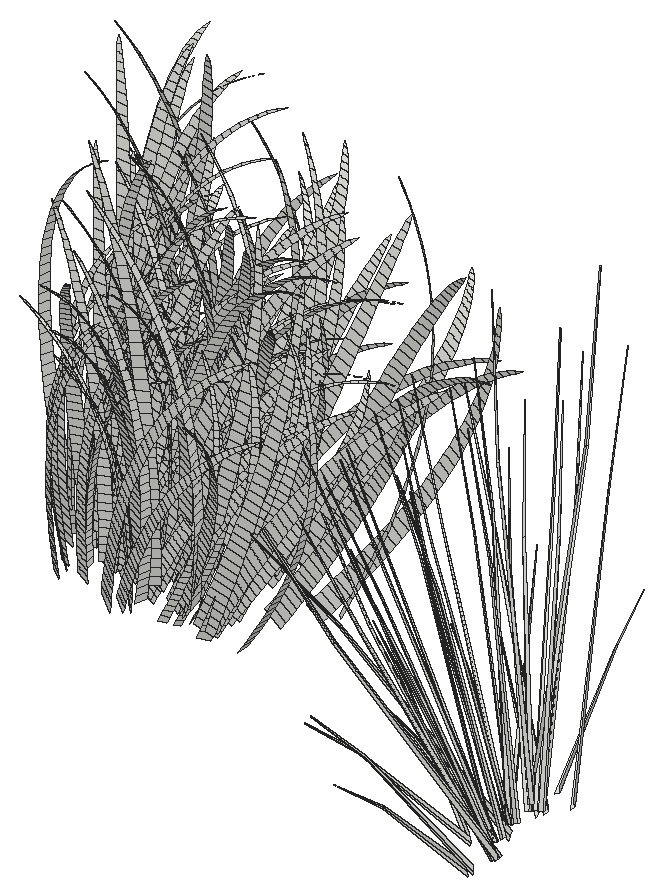
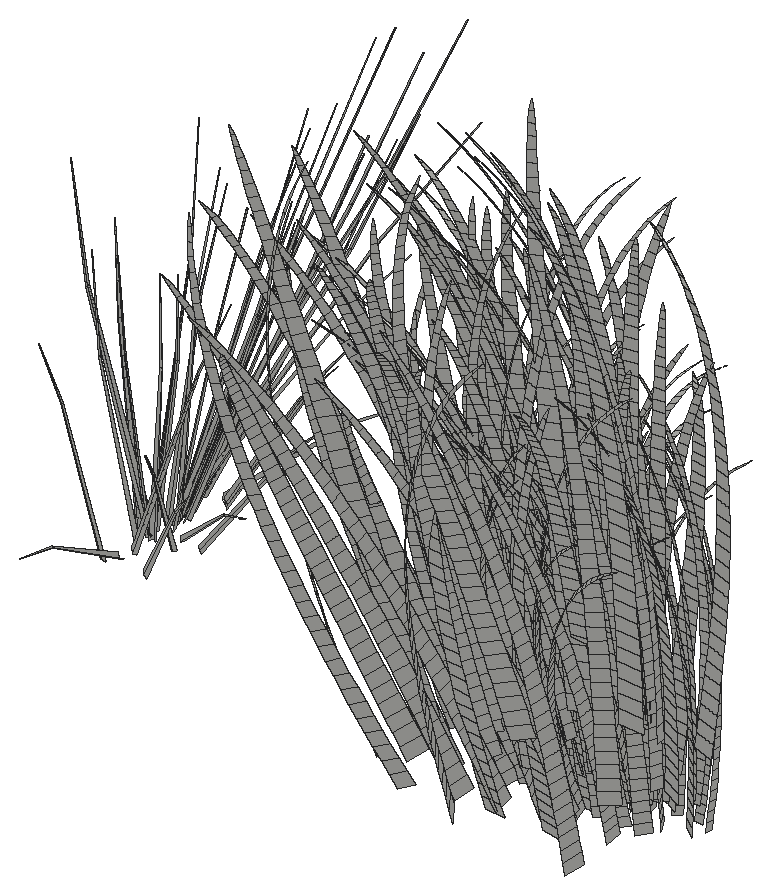
# SketchUp Ruby script. Lengths in inches.
U = 1.inch
M = Sketchup.active_model
def pt(a) = Geom::Point3d.new(a.map { |v| v * U })
def face(e, loops, mat)
  f = e.add_face(loops[0].map { |a| pt(a) })
  loops[1..].each { |l| e.add_face(l.map { |a| pt(a) }).erase! }
  f.material = f.back_material = mat if mat
  f
end
# faces: each face lists its corners as indices into pts; further lists are holes
def faces(e, pts, list, mat = nil) = list.each { |f| face(e, (f[0].is_a?(Array) ? f : [f]).map { |l| l.map { |i| pts[i] } }, mat) }
# xy, xz, yz: faces in a plane at the given z, y or x. An outline is a flat list of corners, or four numbers for a rectangle; further outlines are holes
def ring(l) = l.size == 4 ? [[l[0], l[1]], [l[2], l[1]], [l[2], l[3]], [l[0], l[3]]] : l.each_slice(2).to_a
def flat(e, list, mat, &to3) = list.each { |f| face(e, (f[0].is_a?(Array) ? f : [f]).map { |l| ring(l).map { |u, v| to3.(u, v) } }, mat) }
def xy(e, z, list, mat = nil) = flat(e, list, mat) { |x, y| [x, y, z] }
def xz(e, y, list, mat = nil) = flat(e, list, mat) { |x, z| [x, y, z] }
def yz(e, x, list, mat = nil) = flat(e, list, mat) { |y, z| [x, y, z] }
def lines(e, pts, list) = list.each { |a, b| e.add_line(pt(pts[a]), pt(pts[b])) }
# prism: a flat outline (further loops are holes) pulled along v
def prism(e, loops, v, mat = nil)
  f = face(e, loops, mat); d = Geom::Vector3d.new(v.map { |x| x * U })
  f.pushpull(f.normal.samedirection?(d) ? d.length : -d.length)
end
def box(e, o, s, mat = nil) = prism(e, [[o, [o[0] + s[0], o[1], o[2]], [o[0] + s[0], o[1] + s[1], o[2]], [o[0], o[1] + s[1], o[2]]]], [0, 0, s[2]], mat)
def at(x, y, z, deg = 0) = Geom::Transformation.translation(pt([x, y, z])) * Geom::Transformation.rotation(ORIGIN, Z_AXIS, deg.degrees)
def axes(o, x, y, z) = Geom::Transformation.new([*x, 0, *y, 0, *z, 0, *pt(o).to_a, 1])
def part(name) = M.definitions.add(name)
# library, detail: a bought-in or finely detailed component or shape, given as its bounding box
def library(name, o, s) = part(name).tap { |d| box(d.entities, o, s) }
def detail(e, o, s) = box(e.add_group.entities, o, s)
def put(e, d, t, mat = nil) = e.add_instance(d, t).tap { |i| i.material = mat if mat }
def group(e, t, mat = nil) = e.add_group.tap { |g| g.transformation = t; g.material = mat if mat }.entities
root = M.entities
c1 = part("fur_instance\#8")
p = [[-0.25,1.49,0.03],[0.25,-1.49,-0.03],[0.44,-1.47,1.51],[-0.05,1.47,1.57],[0.65,-1.44,3.05],[0.16,1.45,3.11],
  [0.86,-1.42,4.59],[0.38,1.44,4.65],[1.1,-1.39,6.13],[0.62,1.43,6.18],[1.34,-1.35,7.66],[0.875,1.42,7.72],
  [1.6,-1.32,9.19],[1.14,1.41,9.25],[1.88,-1.28,10.72],[1.43,1.41,10.78],[2.18,-1.24,12.25],[1.73,1.41,12.3],
  [2.49,-1.19,13.77],[2.05,1.41,13.82],[2.83,-1.15,15.29],[2.4,1.41,15.34],[3.18,-1.09,16.8],[2.76,1.42,16.85],
  [3.56,-1.03,18.31],[3.14,1.43,18.35],[3.96,-0.97,19.81],[3.55,1.44,19.85],[4.38,-0.91,21.3],[3.99,1.46,21.35],
  [4.84,-0.83,22.78],[4.45,1.48,22.83],[5.32,-0.76,24.26],[4.93,1.51,24.31],[5.82,-0.67,25.73],[5.45,1.54,25.77],
  [6.36,-0.59,27.18],[6,1.57,27.23],[6.93,-0.49,28.625],[6.58,1.61,28.67],[7.54,-0.39,30.05],[7.19,1.66,30.1],
  [8.18,-0.28,31.47],[7.84,1.71,31.51],[8.85,-0.16,32.86],[8.53,1.77,32.9],[9.57,-0.04,34.24],[9.25,1.83,34.27],
  [10.32,0.09,35.59],[10.02,1.9,35.625],[11.12,0.23,36.92],[10.82,1.97,36.95],[11.95,0.38,38.22],[11.67,2.06,38.25],
  [12.84,0.54,39.49],[12.57,2.14,39.52],[13.76,0.71,40.73],[13.51,2.24,40.76],[14.73,0.89,41.93],[14.49,2.34,41.95],
  [15.75,1.08,43.09],[15.52,2.45,43.11],[16.82,1.28,44.2],[16.6,2.5625,44.23],[17.93,1.5,45.27],[17.73,2.68,45.29],
  [19.08,1.73,46.28],[18.9,2.81,46.3],[20.29,1.97,47.24],[20.125,2.93,47.26],[21.53,2.22,48.13],[21.39,3.0625,48.15],
  [22.82,2.5,48.96],[22.7,3.1875,48.98],[24.14,2.8125,49.72],[24.06,3.3,49.73],[25.48,3.27,50.41]]
faces(c1.entities,p,[[0,1,2,3],[3,2,4,5],[5,4,6,7],[7,6,8,9],[9,8,10,11],[11,10,12,13],[13,12,14,15],[15,14,16,17],
  [17,16,18,19],[19,18,20,21],[21,20,22,23],[23,22,24,25],[25,24,26,27],[27,26,28,29],[29,28,30,31],[31,30,32,33],
  [33,32,34,35],[35,34,36,37],[37,36,38,39],[39,38,40,41],[41,40,42,43],[43,42,44,45],[45,44,46,47],[47,46,48,49],
  [49,48,50,51],[51,50,52,53],[53,52,54,55],[55,54,56,57],[57,56,58,59],[59,58,60,61],[61,60,62,63],[63,62,64,65],
  [65,64,66,67],[67,66,68,69],[69,68,70,71],[71,70,72,73],[73,72,74,75],[75,74,76]])
c2 = part("blade")
p = [[2.15,0.21,22],[0,0.17,0],[0.09,0.45,0],[2.18,0.31,22],[2.29,0.31,22],[0.38,0.45,0],
  [2.48,0.24,33],[2.49,0.24,33],[2.48,0.22,33]]
faces(c2.entities,p,[[0,1,2,3],[4,5,2,3],[6,3,4,7],[8,0,3,6]])
c3 = part("blade with seeds\#1")
put(c3.entities,c2,at(0,0,0))
put(root,c1,axes([173.87,43.59,16.78],[0.3868,0.02345,0.03078],[-0.124,0.10185,-0.10704],[-0.07471,0.00245,0.39218]))
put(root,c1,axes([173.18,43.33,21.52],[0.43328,-0.09632,-0.05486],[0.35647,0.08162,0.1669],[-0.08185,-0.06828,0.53142]))
put(root,c1,axes([174.91,41.51,16.04],[0.3182,0.02541,0.09927],[-0.17585,0.08014,0.05641],[-0.07189,-0.04163,0.34755]))
put(root,c1,axes([179.21,42.91,16.11],[-0.26003,0.0747,-0.01605],[-0.27089,-0.06034,0.10035],[0.05419,-0.00146,0.36045]))
put(root,c1,axes([178.13,41.52,17.22],[-0.18331,0.07729,0.21554],[-0.40147,-0.03636,-0.02445],[0.06494,-0.07386,0.38321]))
put(root,c1,axes([179.87,41.28,15.9375],[-0.39365,0.00146,0.10745],[-0.03589,-0.08049,-0.16462],[0.09278,-0.0639,0.34927]))
put(root,c1,axes([174.18,44.63,19.15],[0.39098,0.0662,-0.03361],[-0.2925,0.10549,-0.12715],[-0.06392,0.0054,0.46798]))
put(root,c1,axes([176.02,42.44,19.22],[0.09644,-0.10652,-0.14889],[0.48091,0.00821,0.03345],[-0.01642,-0.06341,0.45978]))
put(root,c1,axes([174.91,41.83,17.28],[0.34843,0.03828,0.10845],[-0.2361,0.08663,0.07489],[-0.0614,-0.05122,0.39865]))
put(root,c1,axes([177.99,43.69,21.73],[-0.04023,0.1359,0.05604],[-0.56359,0.00089,0.03258],[0.02324,-0.04497,0.55444]))
put(root,c1,axes([175.1,41.28,15.99],[0.37036,-0.00789,0.09527],[-0.06926,0.07694,0.16213],[-0.08348,-0.05968,0.3313]))
put(root,c1,axes([177.42,42.03,18.63],[-0.02474,0.10748,0.14601],[-0.4889,0.00045,0.0409],[0.03862,-0.06244,0.4604]))
put(root,c1,axes([178.53,43.57,19.36],[-0.08585,0.1194,0.00255],[-0.47668,-0.01241,0.04323],[0.03171,-0.0262,0.47718]))
put(root,c1,axes([177.43,43.15,19.35],[0.00743,0.11704,0.02137],[-0.4806,0.01012,0.04491],[0.03344,-0.03278,0.47301]))
put(root,c1,axes([177.06,42.76,17.2],[0.10283,0.09424,-0.02934],[-0.38702,0.0342,0.00026],[-0.00192,-0.015,0.39421]))
put(root,c1,axes([173.875,43.25,18.625],[0.44325,0.01378,0.03894],[-0.10529,0.11313,-0.01664],[-0.05345,-0.02225,0.45082]))
put(root,c1,axes([174.65,41.02,15.42],[0.38165,0.00812,0.0967],[-0.13077,0.07806,0.17346],[-0.05221,-0.06667,0.34902]))
put(root,c1,axes([180.58,44.73,15.37],[-0.39682,0.05407,0.00001],[-0.14979,-0.08823,0.26648],[0.10419,0.03894,0.33892]))
put(root,c1,axes([181.3,45.46,17.51],[-0.48095,0.02794,0.10675],[-0.04773,-0.12201,0.1968],[0.12466,0.01723,0.4389]))
put(root,c1,axes([180.83,42.51,17.77],[-0.42899,-0.01814,0.11625],[0.07503,-0.10666,-0.06158],[0.11661,-0.03633,0.42516]))
put(root,c1,axes([175.72,45.98,23.18],[0.26145,0.12979,-0.04349],[-0.54364,0.07722,-0.0079],[-0.0029,-0.02259,0.59384]))
put(root,c1,axes([180.22,41.06,14.98],[-0.34639,-0.01812,0.09037],[0.04524,-0.07379,-0.15149],[0.11056,-0.0532,0.31576]))
put(root,c1,axes([176.26,44.125,20.55],[0.17418,-0.12594,0.02517],[0.49047,0.0329,-0.02963],[0.00703,-0.0205,0.51235]))
put(root,c1,axes([180.59,41.7,18.06],[-0.38699,-0.07714,-0.06437],[0.35159,-0.0734,-0.25194],[0.12272,-0.08452,0.462]))
put(root,c1,axes([175.84,44.84,16.51],[0.24528,-0.09598,0.1617],[0.37117,0.05209,-0.11468],[-0.0048,0.02754,0.3919]))
put(root,c1,axes([176.22,42.91,17.54],[0.24902,-0.0884,0.02833],[0.33061,0.05438,-0.0118],[-0.0179,-0.01504,0.4078]))
put(root,c1,axes([181.39,44.09,21.17],[-0.4836,-0.06037,0.13492],[0.24695,-0.12356,-0.08931],[0.14971,-0.03767,0.53195]))
put(root,c1,axes([176.53,46.74,18.82],[0.2012,-0.12696,0.22046],[0.50167,0.03853,-0.09696],[-0.00583,0.03346,0.47614]))
put(root,c1,axes([179.38,42.28,16.39],[-0.20329,-0.07557,0.08149],[0.30353,-0.05638,-0.06608],[0.09297,-0.0147,0.35701]))
put(root,c1,axes([177.51,43.04,17.13],[0.10708,0.0959,-0.10596],[-0.38827,0.03586,0.0183],[0.0377,0.00172,0.38456]))
put(root,c1,axes([180.6,41.34,16.9],[-0.3432,-0.0765,-0.07459],[0.35163,-0.06451,-0.23271],[0.11533,-0.07943,0.43417]))
put(root,c1,axes([175.84,42.54,17.01],[0.36393,0.02604,0.01139],[-0.14098,0.09441,-0.02891],[-0.03096,-0.01519,0.38522]))
put(root,c1,axes([180.4375,44.26,15.82],[-0.35276,0.06636,0.01207],[-0.18791,-0.0794,0.2604],[0.14782,0.03047,0.33015]))
put(root,c1,axes([178.6,42.83,16.57],[-0.06056,-0.09523,0.0917],[0.37894,-0.0237,-0.04877],[0.05538,-0.00149,0.36838]))
put(root,c1,axes([176.82,44.14,22.45],[0.21319,0.12584,0.03757],[-0.5414,0.06125,0.05518],[0.02394,-0.04631,0.57097]))
put(root,c1,axes([175.6,43.61,16.52],[0.399,-0.01643,0.04529],[0.04139,0.09756,-0.17419],[-0.04165,0.02519,0.3551]))
put(root,c1,axes([176.61,41.1,15.75],[0.29844,0.03666,0.12007],[-0.24145,0.06247,0.14412],[-0.01396,-0.06488,0.32954]))
put(root,c1,axes([175.37,44.35,19.07],[0.41308,-0.07136,0.08442],[0.24806,0.09913,-0.09648],[-0.03609,0.00646,0.45942]))
put(root,c1,axes([178.26,45.34,19.39],[0.08392,0.12661,-0.13213],[-0.5075,0.03268,0.03746],[0.04815,0.00219,0.49115]))
put(root,c1,axes([181.8,42.8125,18.18],[-0.35421,0.07276,0.12893],[-0.29124,-0.08765,0.05062],[0.12278,-0.03826,0.44767]))
put(root,c1,axes([183.08,45.72,21.29],[-0.50822,-0.05914,0.16088],[0.26318,-0.13542,0.00476],[0.12972,-0.0152,0.55648]))
put(root,c1,axes([179.42,43.74,20.68],[0.02612,0.1296,0.0118],[-0.53066,0.01567,0.05121],[0.03825,-0.03377,0.52318]))
put(root,c1,axes([181.06,41.09,15.72],[-0.34665,0.03766,0.28281],[-0.2966,-0.07324,-0.12549],[0.15318,-0.08977,0.36049]))
put(root,c1,axes([178.11,43.89,22.05],[0.15528,0.1304,0.03251],[-0.55243,0.04732,0.0551],[0.03088,-0.04382,0.56366]))
put(root,c1,axes([180.04,43.95,16.07],[-0.20898,-0.0824,0.18746],[0.34722,-0.06501,-0.01016],[0.10453,0.01445,0.36802]))
put(root,c1,axes([176.22,41.99,16.82],[0.37924,-0.02367,0.00941],[0.05552,0.08897,0.04526],[-0.02563,-0.0313,0.37636]))
put(root,c1,axes([179.16,41.89,16.54],[-0.0973,-0.0872,-0.02774],[0.35951,-0.02338,-0.11019],[0.09232,-0.03585,0.36133]))
put(root,c1,axes([179,42.59,16.48],[0.02752,0.09542,-0.07338],[-0.37422,0.01455,0.07284],[0.07104,-0.00536,0.36252]))
put(root,c1,axes([173.99,45.76,22.99],[0.58805,-0.03865,0.01795],[0.09936,0.14447,-0.04041],[-0.02579,-0.02167,0.5876]))
put(root,c1,axes([178.87,42.01,16.91],[-0.00466,0.09305,0.05851],[-0.38392,-0.00135,0.10148],[0.09517,-0.03696,0.37249]))
put(root,c1,axes([176.79,41.53,16.45],[0.34452,-0.04366,-0.04731],[0.16007,0.07028,0.10831],[-0.01271,-0.04911,0.3561]))
put(root,c1,axes([181.05,41.9,15.94],[-0.33959,-0.02161,0.16129],[0.05445,-0.08788,-0.07973],[0.16742,-0.03443,0.33197]))
put(root,c1,axes([176.51,42.19,17.27],[0.37389,-0.04384,-0.01604],[0.14616,0.08522,0.04602],[-0.01175,-0.03392,0.39343]))
put(root,c1,axes([182.08,42.98,15.46],[-0.35465,0.03179,0.12412],[-0.08422,-0.0944,0.12866],[0.14822,-0.00049,0.34485]))
put(root,c1,axes([176.58,42.93,18.67],[0.28277,-0.09216,-0.0293],[0.35374,0.06329,-0.03099],[0.03198,-0.02663,0.44612]))
put(root,c1,axes([181.62,41.28,16.91],[-0.23365,0.08018,0.37739],[-0.5281,-0.04795,-0.04906],[0.12206,-0.1166,0.44118]))
put(root,c1,axes([181.47,45.32,14.72],[-0.24838,-0.07552,0.26827],[0.36264,-0.07613,0.06552],[0.10797,0.04035,0.35122]))
put(root,c1,axes([177.51,42.49,16.78],[0.31248,0.04845,-0.02906],[-0.22065,0.08233,-0.00534],[0.01159,-0.01612,0.37663]))
put(root,c1,axes([179.18,44.03,15.98],[0.02256,-0.10291,0.16613],[0.40828,-0.00696,-0.08216],[0.0702,0.01977,0.36521]))
put(root,c1,axes([181.11,42.56,16.15],[-0.29666,-0.04989,0.17471],[0.19623,-0.0852,-0.04047],[0.16374,-0.00882,0.3424]))
put(root,c1,axes([179.03,45.94,23.03],[-0.03607,-0.15174,0.11498],[0.59448,-0.02115,-0.11709],[0.11275,-0.0085,0.57541]))
put(root,c1,axes([177.24,43.88,22.48],[0.37939,0.0996,0.02895],[-0.4487,0.09947,0.0626],[0.0152,-0.04823,0.57611]))
put(root,c1,axes([178.41,43.27,15.38],[0.1407,-0.08863,0.11524],[0.33667,0.02483,-0.11863],[0.06264,0.01764,0.32589]))
put(root,c1,axes([177.15,45.68,16.15],[0.3727,-0.07301,0.16563],[0.28524,0.07874,-0.23301],[-0.00162,0.05084,0.36457]))
put(root,c1,axes([176.78,44.3,16.9],[0.43051,-0.02394,0.0206],[0.06045,0.10399,-0.19261],[-0.00469,0.02691,0.38296]))
put(root,c1,axes([178.24,41.6,16.8],[0.22861,0.07303,0.05639],[-0.33302,0.05317,0.11142],[0.05286,-0.04974,0.38225]))
put(root,c1,axes([179.35,43.29,20.28],[0.01264,0.12288,0.07226],[-0.50693,0.00277,0.13679],[0.12569,-0.04881,0.49196]))
put(root,c1,axes([177.16,44.03,20.13],[0.34488,-0.10012,0.002],[0.37363,0.0781,-0.03923],[0.0154,-0.02142,0.50061]))
put(root,c1,axes([178.18,42.6,16.96],[0.27118,-0.07576,-0.00645],[0.28316,0.06173,-0.03098],[0.01761,-0.01788,0.38612]))
put(root,c1,axes([176.8,49.28,16.01],[0.42291,-0.09938,0.23214],[0.39627,0.08778,-0.26596],[-0.002,0.06278,0.45019]))
put(root,c1,axes([183.08,43.41,16.97],[-0.4106,-0.00543,0.20139],[0.04205,-0.11444,0.05244],[0.19001,-0.01023,0.39734]))
put(root,c1,axes([182.77,44.35,15.18],[-0.36895,0.05606,0.09915],[-0.13288,-0.09289,0.24927],[0.19273,0.02154,0.33775]))
put(root,c1,axes([183.29,42.07,17.9375],[-0.37153,-0.08434,-0.02213],[0.34879,-0.07192,-0.25637],[0.16129,-0.07761,0.46063]))
put(root,c1,axes([184.86,41.54,16.58],[-0.50186,0.02355,0.30155],[-0.25313,-0.0987,-0.23318],[0.18872,-0.1106,0.44413]))
put(root,c1,axes([183.2,44.1,15.52],[-0.39061,0.03518,0.15062],[-0.0516,-0.10317,0.22352],[0.19364,0.02164,0.33934]))
put(root,c1,axes([176.03,43.88,21.7],[0.55785,-0.00791,-0.01628],[-0.01652,0.13309,0.06461],[0.0048,-0.04675,0.54689]))
put(root,c1,axes([183.28,43.63,18.64],[-0.4509,0.00616,0.22882],[-0.0181,-0.12521,0.04122],[0.22278,-0.02264,0.43901]))
put(root,c1,axes([183.67,43.38,21.2],[-0.48309,-0.08026,0.09146],[0.28649,-0.10364,-0.27324],[0.21845,-0.07803,0.52044]))
put(root,c1,axes([176.04,44.3,22.84],[0.5666,0.02979,-0.00978],[-0.17183,0.13867,0.06881],[0.01531,-0.0486,0.58051]))
put(root,c1,axes([185.26,48.55,16.03],[-0.55014,0.02901,0.18365],[0.00085,-0.13945,0.30825],[0.20346,0.04194,0.45443]))
put(root,c1,axes([178.65,42.05,16.51],[0.32227,-0.05147,-0.03571],[0.18703,0.07572,-0.00913],[0.02683,-0.02369,0.36692]))
put(root,c1,axes([177.82,43.03,16.91],[0.37256,-0.04353,-0.00886],[0.13876,0.09121,-0.10577],[0.03721,0.00169,0.3796]))
put(root,c1,axes([182.4,42.46,15.43],[-0.23007,0.07314,0.09888],[-0.26121,-0.06326,0.14962],[0.17184,-0.01746,0.33863]))
put(root,c1,axes([179.48,42.08,18.72],[0.26451,0.09374,0.07646],[-0.42666,0.06178,0.13506],[0.06569,-0.06182,0.47506]))
put(root,c1,axes([180.46,42.72,15.38],[0.0428,-0.09225,0.10006],[0.34352,0.00073,-0.13098],[0.11685,0.00658,0.3208]))
put(root,c1,axes([177.49,43.37,20.22],[0.49662,0.02151,-0.02814],[-0.12608,0.12198,0.04971],[0.02758,-0.03912,0.50329]))
put(root,c1,axes([176.84,42.68,21.14],[0.5576,-0.04981,-0.0814],[0.1812,0.11742,0.16274],[0.01381,-0.07598,0.54958]))
put(root,c1,axes([182.45,41.38,14.68],[-0.22568,0.04158,0.23633],[-0.22234,-0.07345,0.05473],[0.21423,-0.04741,0.28926]))
put(root,c1,axes([183.64,47.1875,16.04],[-0.29108,-0.08992,0.33015],[0.41587,-0.09585,0.02478],[0.18773,0.0387,0.41931]))
put(root,c1,axes([181.02,43.75,19.21],[0.11851,0.11876,-0.04717],[-0.4673,0.03445,0.1331],[0.13073,-0.02639,0.47242]))
put(root,c1,axes([183.37,44.77,17.67],[-0.24392,-0.10076,0.20467],[0.39271,-0.0762,-0.09756],[0.18799,-0.00063,0.43735]))
put(root,c1,axes([184.43,46.6,18.75],[-0.24714,0.13384,-0.07511],[-0.47681,-0.05071,0.24443],[0.18128,0.01021,0.49768]))
put(root,c1,axes([178.84,41.87,16.46],[0.35258,0.02235,-0.0802],[-0.09139,0.08541,0.07692],[0.09028,-0.03506,0.35336]))
put(root,c1,axes([178.76,42.96,17.83],[0.36096,0.04893,-0.11793],[-0.21378,0.09664,0.00322],[0.09509,-0.01114,0.4079]))
put(root,c1,axes([183.27,41.76,14.52],[-0.26142,0.03054,0.23438],[-0.15684,-0.08384,0.05286],[0.22838,-0.03655,0.28923]))
put(root,c1,axes([180.29,42.68,17.45],[0.17357,-0.09808,-0.04046],[0.37671,0.04122,-0.11456],[0.11247,-0.02271,0.40645]))
put(root,c1,axes([183.38,41.65,15.75],[-0.28567,-0.07961,0.0175],[0.26475,-0.04599,-0.28592],[0.22394,-0.06695,0.33858]))
put(root,c1,axes([185.8125,43.55,18.77],[-0.4701,0.02698,0.25684],[-0.14161,-0.12634,-0.00193],[0.239,-0.04915,0.4739]))
put(root,c1,axes([182.26,46.6,20.58],[-0.05466,0.14737,-0.16504],[-0.55037,0.00251,0.2052],[0.18669,0.01051,0.51252]))
put(root,c1,axes([182.86,42.71,16.5625],[-0.12139,0.09912,0.07892],[-0.3681,-0.03704,0.18622],[0.19491,-0.0294,0.37749]))
put(root,c1,axes([182.53,43.6875,20.7],[-0.05395,-0.13445,-0.03502],[0.54148,-0.01404,-0.1606],[0.1457,-0.0454,0.53123]))
put(root,c1,axes([180.44,42.69,17.07],[0.25328,0.0781,-0.08233],[-0.31324,0.06765,0.08453],[0.10923,-0.02205,0.39474]))
put(root,c1,axes([183.94,42.25,14.76],[-0.30953,0.00742,0.24868],[-0.05422,-0.09712,0.02506],[0.24517,-0.02632,0.30384]))
put(root,c1,axes([178.6875,40.69,14.96],[0.51274,0.02643,0.07535],[-0.18873,0.07879,0.34618],[0.04747,-0.11121,0.40935]))
put(root,c1,axes([180.9375,41.875,15.62],[0.11275,0.08491,-0.04547],[-0.30687,0.02749,0.16442],[0.16441,-0.0248,0.31841]))
put(root,c1,axes([179.61,40.87,15.04],[0.37669,0.0324,0.02789],[-0.15541,0.05741,0.26709],[0.08613,-0.08228,0.31131]))
put(root,c1,axes([184.32,42.18,15.29],[-0.32481,0.01159,0.26858],[-0.10314,-0.09907,-0.00298],[0.25531,-0.04086,0.32333]))
put(root,c1,axes([184.95,42.32,15.12],[-0.34499,-0.02738,0.25117],[0.02857,-0.09755,-0.10655],[0.25933,-0.0415,0.32843]))
put(root,c1,axes([183.92,46.32,21.08],[-0.15452,0.1484,-0.07681],[-0.53114,-0.02876,0.26019],[0.22493,-0.00075,0.52331]))
put(root,c1,axes([183.9,43.64,19.91],[-0.05123,-0.13135,-0.03464],[0.52898,-0.01334,-0.15675],[0.1423,-0.04434,0.51883]))
put(root,c1,axes([179.2,42.71,20.26],[0.54003,0.00824,-0.06609],[-0.05181,0.12104,0.15416],[0.07099,-0.06681,0.51339]))
put(root,c1,axes([179.78,45.75,16.57],[0.38423,-0.08292,0.07496],[0.27259,0.07958,-0.28633],[0.11572,0.04325,0.37644]))
put(root,c1,axes([180.94,41.65,16],[0.2441,0.07222,-0.04355],[-0.26394,0.05308,0.1817],[0.16084,-0.04366,0.34094]))
put(root,c1,axes([179.82,43.39,20.92],[0.42795,0.07728,-0.03537],[-0.32717,0.10078,0.16162],[0.11703,-0.05783,0.5184]))
put(root,c1,axes([185.4375,41.6,14.43],[-0.23369,0.05664,0.2885],[-0.32329,-0.07522,0.05329],[0.22936,-0.06857,0.34676]))
put(root,c1,axes([184.59,42.8,15.66],[-0.24319,0.0675,0.20698],[-0.24252,-0.08231,0.17828],[0.26796,-0.02877,0.33209]))
put(root,c1,axes([184.03,41.79,17.11],[-0.09117,0.08927,0.31255],[-0.47937,-0.04642,0.14327],[0.22373,-0.09133,0.40321]))
put(root,c1,axes([180.42,43.83,18.09],[0.43816,-0.04115,-0.06829],[0.12625,0.10984,-0.10547],[0.08633,-0.00651,0.44055]))
put(root,c1,axes([181.11,43.62,21.92],[0.28774,-0.11989,-0.16846],[0.50898,0.06802,-0.06219],[0.12703,-0.06277,0.56267]))
put(root,c1,axes([181.83,42.08,18.24],[0.24015,0.0994,0.09665],[-0.43311,0.04149,0.23064],[0.15674,-0.07542,0.44765]))
put(root,c1,axes([183.61,43.21,19.68],[-0.08653,-0.12451,-0.08606],[0.49279,-0.00764,-0.24538],[0.22385,-0.06076,0.47449]))
put(root,c1,axes([181.57,43.01,20.81],[0.33121,-0.10708,-0.17554],[0.46429,0.07502,-0.01094],[0.1013,-0.06638,0.54407]))
put(root,c1,axes([181.73,41.79,16.87],[0.25074,0.08698,0.01816],[-0.3444,0.04816,0.2178],[0.16569,-0.05919,0.39475]))
put(root,c1,axes([179.48,44.05,20.15],[0.49916,0.00373,-0.14036],[-0.03985,0.12918,-0.03133],[0.12743,-0.02015,0.48937]))
put(root,c1,axes([180.6,43.21,18.11],[0.42952,-0.03052,-0.12246],[0.10448,0.1092,-0.04206],[0.11987,-0.0242,0.43318]))
put(root,c1,axes([187.16,44.125,19.21],[-0.32096,0.10523,0.184],[-0.3983,-0.0918,0.19336],[0.25723,-0.0388,0.49819]))
put(root,c1,axes([181.3125,43.69,21.6],[0.36404,-0.10367,-0.1727],[0.44027,0.08598,-0.03094],[0.12412,-0.06133,0.54977]))
put(root,c1,axes([185.61,44.22,14.99],[-0.19157,-0.09107,0.25878],[0.34369,-0.07171,-0.11605],[0.23799,0.01076,0.35443]))
put(root,c1,axes([185.73,41.875,14.8],[-0.14451,0.08142,0.23663],[-0.35536,-0.06178,0.17404],[0.25941,-0.05741,0.35026]))
put(root,c1,axes([184.91,43.17,15.98],[-0.14974,-0.10284,0.16036],[0.32665,-0.04744,-0.23161],[0.27394,-0.016,0.34581]))
put(root,c1,axes([180.83,44.43,20.15],[0.47366,-0.05752,-0.11313],[0.19907,0.11948,-0.09473],[0.13075,-0.02068,0.50211]))
put(root,c1,axes([184.33,44.36,19.8],[0.02844,0.13663,-0.04942],[-0.49209,0.00914,0.24911],[0.24334,-0.02473,0.47953]))
put(root,c1,axes([181.87,42.19,19.43],[0.44201,0.08093,0.05798],[-0.36622,0.08436,0.27952],[0.13473,-0.09279,0.5072]))
put(root,c1,axes([182.96,41.68,15.81],[0.30391,0.0709,-0.02798],[-0.26837,0.06266,0.20611],[0.15769,-0.05633,0.37569]))
put(root,c1,axes([181.92,45.36,19.54],[0.31281,-0.11582,0.02754],[0.4011,0.07043,-0.24062],[0.1717,0.00967,0.47137]))
put(root,c1,axes([185.57,41.43,15.16],[-0.00768,0.09583,0.28318],[-0.48756,-0.03041,0.19456],[0.22357,-0.09127,0.40293]))
put(root,c1,axes([186.74,43.5,18.0625],[-0.11603,0.12105,0.13085],[-0.47114,-0.04061,0.21751],[0.2362,-0.04858,0.46834]))
put(root,c1,axes([185.79,43.1875,15.3],[-0.12105,0.10671,0.04707],[-0.33828,-0.0379,0.2777],[0.2739,-0.016,0.34577]))
put(root,c1,axes([182.22,43.03,17.9],[0.45,0.00061,-0.13289],[-0.01034,0.11399,0.01813],[0.1241,-0.03123,0.44096]))
put(root,c1,axes([188.2,41.92,14.57],[-0.3444,0.00645,0.39598],[-0.23551,-0.10237,-0.1009],[0.32539,-0.08613,0.32529]))
put(root,c1,axes([183.17,47.1,16.61],[0.40477,-0.09993,0.0388],[0.3095,0.08612,-0.33005],[0.18844,0.03884,0.42089]))
put(root,c1,axes([188.54,47.375,17.8],[-0.1875,0.14787,-0.09777],[-0.47837,-0.0323,0.35719],[0.31076,0.01405,0.46282]))
put(root,c1,axes([187.34,43.37,18.99],[0.08595,0.13269,0.09474],[-0.52589,0.00657,0.26023],[0.2384,-0.06471,0.50535]))
put(root,c1,axes([192.1,46.34,16.23],[-0.48064,-0.00945,0.35551],[0.07484,-0.14996,0.09525],[0.34037,-0.00309,0.45605]))
put(root,c1,axes([188.56,44.32,15.7],[-0.10846,-0.12432,0.13782],[0.39469,-0.03448,-0.28978],[0.31205,-0.01822,0.39392]))
put(root,c1,axes([185.78,47.01,16.3],[0.29244,-0.12451,0.07265],[0.4005,0.05762,-0.33138],[0.24372,0.02724,0.42711]))
put(root,c1,axes([185.93,41.58,15.76],[0.36607,0.09239,0.0562],[-0.35794,0.05108,0.35634],[0.23474,-0.09583,0.42306]))
put(root,c1,axes([188.93,46.12,19.15],[0.08159,-0.15087,0.05653],[0.53987,0.01442,-0.26943],[0.25135,-0.01354,0.52561]))
put(root,c1,axes([189.67,46.88,15.33],[-0.15503,-0.11331,0.38202],[0.40816,-0.08401,-0.19365],[0.36196,0.02671,0.36052]))
put(root,c1,axes([187.78,44.83,18.64],[0.24875,-0.12362,-0.09554],[0.44274,0.06799,-0.24359],[0.25071,-0.02548,0.49405]))
put(root,c3,axes([215.54,36.28,15.19],[0.24703,-0.23521,1.33979],[0.20797,1.08685,0.10833],[-0.38782,0.24564,0.57275]))
put(root,c3,axes([213.91,34.49,15.85],[-0.10788,0.15738,1.36768],[0.06839,1.05028,-0.2163],[-0.25802,0.16762,0.10969]))
put(root,c3,axes([215.73,33.38,16.06],[-0.62562,0.4911,-0.55542],[-0.34866,-1.01092,0.06703],[-0.30228,0.11484,0.78569]))
put(root,c3,axes([214.68,29.99,15.84],[0.05877,0.1045,1.38675],[-0.19828,1.02381,-0.13103],[-0.25647,0.03706,0.24541]))
put(root,c3,axes([215.23,29.77,15.85],[-0.15313,0.00993,1.36768],[-0.44257,0.8389,-0.2163],[-0.26828,-0.1297,0.10969]))
put(root,c3,axes([216.34,31.34,16.06],[-0.71171,-0.02677,-0.55542],[0.0478,-1.12742,0.06703],[-0.30151,-0.11898,0.78569]))
put(root,c3,axes([215.98,32.61,15.19],[0.26446,0.19158,1.33979],[-0.54729,0.80372,0.10833],[-0.3411,-0.36257,0.57275]))
put(root,c3,axes([215.2,33.29,15.7],[-0.59169,-0.3102,-0.27686],[0.17258,-0.905,0.35743],[-0.23822,0.08298,0.68391]))
put(root,c3,axes([213.95,33.125,14.32],[0.44866,-0.132,0.89796],[-0.2485,0.73224,0.65976],[-0.22973,-0.07879,0.19778]))
put(root,c3,axes([215.6,33.75,15.82],[-0.19288,1.01147,-0.39948],[-0.6613,-0.3467,-0.30943],[-0.26625,0.09275,0.76437]))
put(root,c3,axes([213.55,35.5625,15.84],[0.09222,0.0192,1.38675],[0.3347,0.94674,-0.13103],[-0.17109,0.2786,0.24541]))
put(root,c3,axes([216.1,31.57,15.82],[-0.51698,0.73658,-0.39948],[-0.45276,-0.77811,-0.30943],[-0.26267,-0.11207,0.76437]))
put(root,c3,axes([215.57,32.89,16.1],[0.35822,1.00689,-0.09507],[-0.63579,0.49481,-0.52766],[-0.26792,0.13285,0.80177]))
put(root,c3,axes([215.1875,35.77,16.14],[-0.19776,-1.14621,0.42031],[0.77577,-0.19893,0.34656],[-0.22864,0.26957,0.86972]))
put(root,c3,axes([214.49,36.89,14.32],[0.26779,-0.53674,0.89796],[0.16098,0.78168,0.65976],[-0.20581,0.16725,0.19778]))
put(root,c3,axes([215.33,33.18,15.86],[0.20115,-1.01389,0.37528],[0.6613,0.3467,0.30943],[-0.26006,0.06093,0.77654]))
put(root,c3,axes([216.375,30.8,16.1],[-0.03812,1.13085,-0.09507],[-0.7218,-0.03091,-0.52766],[-0.27799,-0.07855,0.80177]))
put(root,c3,axes([215.91,35.6,16.06],[-0.3719,0.87738,-0.55542],[-0.65169,-0.62354,0.06703],[-0.22205,0.31788,0.78569]))
put(root,c3,axes([215.28,32.91,15.86],[-0.26149,-0.75819,0.05027],[0.47684,-0.37111,0.39574],[-0.2102,0.07322,0.60345]))
put(root,c3,axes([215.41,35.9,15.7],[-0.61974,0.15892,-0.27686],[-0.16365,-0.90846,0.35743],[-0.1776,0.24401,0.68391]))
put(root,c3,axes([215.91,30.875,15.7],[-0.4051,-0.6962,-0.27686],[0.46256,-0.65905,0.35743],[-0.23502,-0.10028,0.68391]))
put(root,c3,axes([215.36,35.51,15.86],[-0.48877,-0.46765,0.05027],[0.28456,-0.66596,0.39574],[-0.1567,0.2153,0.60345]))
put(root,c3,axes([216.31,37.85,15.19],[0.13256,-0.3822,1.33979],[0.55613,0.79096,0.10833],[-0.25088,0.49297,0.57275]))
put(root,c3,axes([215.82,33.19,16.11],[0.59169,0.3102,0.27686],[-0.17258,0.905,-0.35743],[-0.23822,0.08298,0.68391]))
put(root,c3,axes([215.31,35.3,16.41],[0.73762,0.68672,-0.10647],[-0.42495,0.99449,-0.59098],[-0.2084,0.34569,0.89798]))
put(root,c3,axes([215.92,36.01,15.82],[0.1829,1.01534,-0.39948],[-0.69265,0.17761,-0.30943],[-0.19849,0.27272,0.76437]))
put(root,c3,axes([216.07,30.875,15.86],[0.52497,-0.7327,0.37528],[0.45276,0.77811,0.30943],[-0.2463,-0.13515,0.77654]))
put(root,c3,axes([216.12,30.61,15.86],[0.03585,-0.84557,0.05027],[0.54135,0.02318,0.39574],[-0.20737,-0.08848,0.60345]))
put(root,c3,axes([216.49,31.24,16.11],[0.4051,0.6962,0.27686],[-0.46256,0.65905,-0.35743],[-0.23502,-0.10028,0.68391]))
put(root,c3,axes([217.29,30.04,15.82],[-0.70255,0.26433,-0.39948],[-0.1229,-1.00103,-0.30943],[-0.1887,-0.28686,0.76437]))
put(root,c3,axes([217.58,30.01,16.06],[-0.60709,-0.53747,-0.55542],[0.43145,-0.94184,0.06703],[-0.21995,-0.32091,0.78569]))
put(root,c3,axes([215.09,37.93,15.85],[-0.00543,0.22139,1.36768],[0.5431,0.70483,-0.2163],[-0.11097,0.37607,0.10969]))
put(root,c3,axes([217.8,29.57,16.1],[-0.42425,0.9518,-0.09507],[-0.6144,-0.54834,-0.52766],[-0.21357,-0.26891,0.80177]))
put(root,c3,axes([215.92,35.36,16.11],[0.61974,-0.15892,0.27686],[0.16365,0.90846,-0.35743],[-0.1776,0.24401,0.68391]))
put(root,c3,axes([217.61,27.22,15.84],[-0.00584,0.13439,1.38675],[-0.62613,0.55808,-0.13103],[-0.20587,-0.22412,0.24541]))
put(root,c3,axes([215.9,28.81,14.32],[0.39167,0.34272,0.89796],[-0.52622,0.29459,0.65976],[-0.13186,-0.28307,0.19778]))
